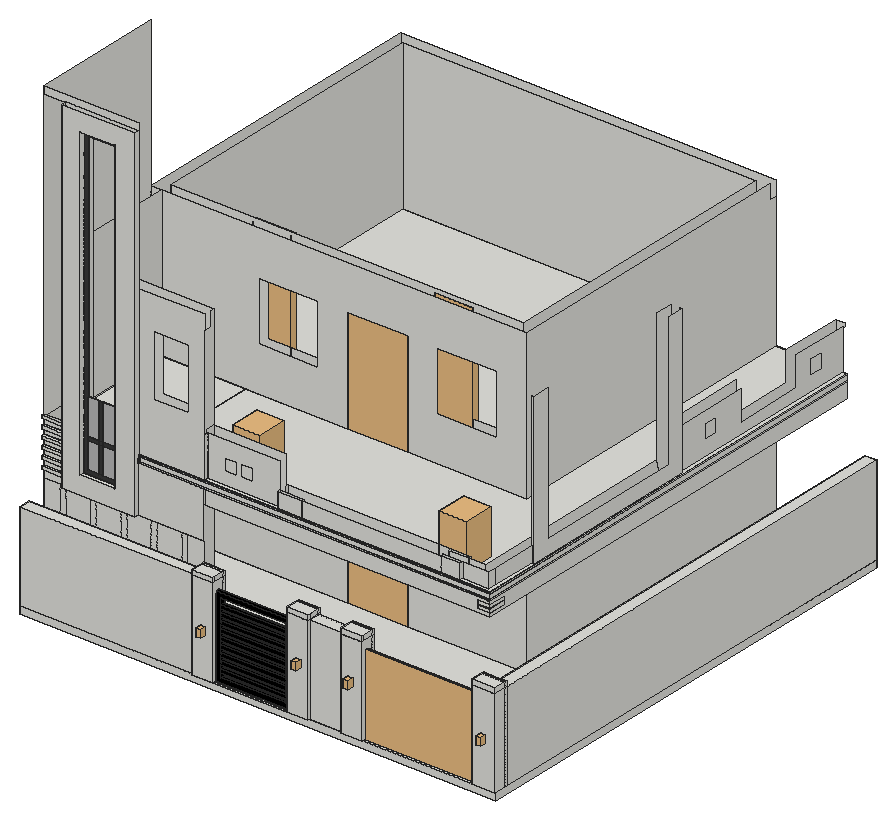
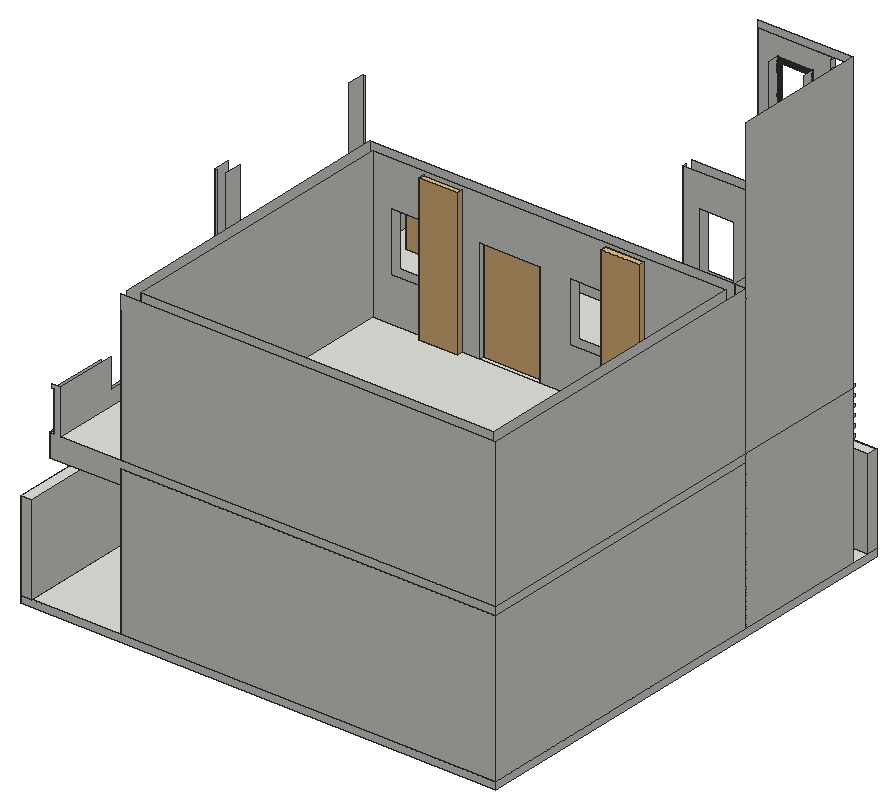
# SketchUp Ruby script. Lengths in inches.
U = 1.inch
M = Sketchup.active_model
def pt(a) = Geom::Point3d.new(a.map { |v| v * U })
def face(e, loops, mat)
  f = e.add_face(loops[0].map { |a| pt(a) })
  loops[1..].each { |l| e.add_face(l.map { |a| pt(a) }).erase! }
  f.material = f.back_material = mat if mat
  f
end
# faces: each face lists its corners as indices into pts; further lists are holes
def faces(e, pts, list, mat = nil) = list.each { |f| face(e, (f[0].is_a?(Array) ? f : [f]).map { |l| l.map { |i| pts[i] } }, mat) }
# xy, xz, yz: faces in a plane at the given z, y or x. An outline is a flat list of corners, or four numbers for a rectangle; further outlines are holes
def ring(l) = l.size == 4 ? [[l[0], l[1]], [l[2], l[1]], [l[2], l[3]], [l[0], l[3]]] : l.each_slice(2).to_a
def flat(e, list, mat, &to3) = list.each { |f| face(e, (f[0].is_a?(Array) ? f : [f]).map { |l| ring(l).map { |u, v| to3.(u, v) } }, mat) }
def xy(e, z, list, mat = nil) = flat(e, list, mat) { |x, y| [x, y, z] }
def xz(e, y, list, mat = nil) = flat(e, list, mat) { |x, z| [x, y, z] }
def yz(e, x, list, mat = nil) = flat(e, list, mat) { |y, z| [x, y, z] }
def lines(e, pts, list) = list.each { |a, b| e.add_line(pt(pts[a]), pt(pts[b])) }
# prism: a flat outline (further loops are holes) pulled along v
def prism(e, loops, v, mat = nil)
  f = face(e, loops, mat); d = Geom::Vector3d.new(v.map { |x| x * U })
  f.pushpull(f.normal.samedirection?(d) ? d.length : -d.length)
end
def box(e, o, s, mat = nil) = prism(e, [[o, [o[0] + s[0], o[1], o[2]], [o[0] + s[0], o[1] + s[1], o[2]], [o[0], o[1] + s[1], o[2]]]], [0, 0, s[2]], mat)
def at(x, y, z, deg = 0) = Geom::Transformation.translation(pt([x, y, z])) * Geom::Transformation.rotation(ORIGIN, Z_AXIS, deg.degrees)
def axes(o, x, y, z) = Geom::Transformation.new([*x, 0, *y, 0, *z, 0, *pt(o).to_a, 1])
def part(name) = M.definitions.add(name)
# library, detail: a bought-in or finely detailed component or shape, given as its bounding box
def library(name, o, s) = part(name).tap { |d| box(d.entities, o, s) }
def detail(e, o, s) = box(e.add_group.entities, o, s)
def put(e, d, t, mat = nil) = e.add_instance(d, t).tap { |i| i.material = mat if mat }
def group(e, t, mat = nil) = e.add_group.tap { |g| g.transformation = t; g.material = mat if mat }.entities
root = M.entities
M.materials.add("[Color M07]").color = [58, 58, 58]
M.materials.add("[Color M09]").color = [0, 0, 0]
M.materials.add("[Mirror 01]").color = [185, 185, 185]
c1 = library("Modern Gate 1",[0,0,0],[118.11,1.97,78.74])
c2 = library("Curtains 004",[-15.59,-2.26,0],[31.18,4.52,116.91])
c3 = library("Door 243 053",[-21.6,-2.79,-0.07],[43.2,5.58,82.64])
c4 = library("Lamp Wall Outdoor 94-02",[-1.89,-4.65,-3.17],[3.78,4.65,6.35])
c5 = library("Window 46-10",[-43.56,-2.12,0],[87.13,4.27,82.67])
c6 = library("Ficus elastica Belize 002",[-7.92,-8.8125,0.01],[22.14,24.73,36.43])
xy(root,-6,[[7.9375,1.1875,391.9375,385.1875]])
xy(root,0,[[147.375,0,164.42,1.1875],[164.42,0,224.25,1.1875],[224.25,0,241.3,1.1875],[267.83,0,284.875,1.1875],[373.38,0,391.9375,1.1875],
  [7.9375,1.1875,147.375,10.1875],[147.375,1.1875,164.42,10.1875],[164.42,1.1875,224.25,3.2],[224.25,1.1875,241.3,10.1875],[241.3,1.1875,267.83,10.1875],
  [267.83,1.1875,284.875,10.1875],[284.875,1.1875,373.38,10.1875],[373.38,1.1875,391.9375,10.1875],[164.42,3.2,224.25,6.14],[164.42,6.14,224.25,10.1875],
  [7.9375,10.1875,147.375,10.1875,147.375,11.875,164.42,11.875,164.42,10.1875,224.25,10.1875,224.25,11.875,241.3,11.875,241.3,10.1875,267.83,10.1875,267.83,11.875,284.875,11.875,284.875,10.1875,373.38,10.1875,373.38,11.875,382.9375,11.875,382.9375,385.1875,310.9375,385.1875,310.9375,133.1875,214.9375,133.1875,214.9375,142.1875,166.9375,142.1875,166.9375,133.1875,16.9375,133.1875,16.9375,34.1875,137.39,34.1875,137.39,25.1875,7.9375,25.1875],[147.375,10.1875,164.42,11.875],[224.25,10.1875,241.3,11.875],[267.83,10.1875,284.875,11.875],[373.38,10.1875,382.9375,11.875],
  [382.9375,10.1875,391.9375,11.875],[382.9375,11.875,391.9375,385.1875],[7.9375,25.1875,16.9375,133.1875],[16.9375,25.1875,137.39,34.1875],[7.9375,133.1875,166.9375,133.1875,166.9375,142.1875,16.9375,142.1875,16.9375,376.1875,301.9375,376.1875,301.9375,142.1875,214.9375,142.1875,214.9375,133.1875,310.9375,133.1875,310.9375,385.1875,7.9375,385.1875],
  [16.9375,142.1875,301.9375,376.1875],[16.9375,142.1875,301.9375,376.1875]])
xy(root,3.64,[[168.07,3.2,220.61,6.14]],"[Color M09]")
xy(root,6.82,[[168.07,3.2,220.61,6.14]],"[Color M09]")
xy(root,9.91,[[168.07,3.2,220.61,6.14]],"[Color M09]")
xy(root,12.64,[[168.07,3.2,220.61,6.14]],"[Color M09]")
xy(root,15.73,[[168.07,3.2,220.61,6.14]],"[Color M09]")
xy(root,18.46,[[168.07,3.2,220.61,6.14]],"[Color M09]")
xy(root,21.55,[[168.07,3.2,220.61,6.14]],"[Color M09]")
xy(root,24.29,[[168.07,3.2,220.61,6.14]],"[Color M09]")
xy(root,27.37,[[168.07,3.2,220.61,6.14]],"[Color M09]")
xy(root,30.11,[[168.07,3.2,220.61,6.14]],"[Color M09]")
xy(root,33.1875,[[168.07,3.2,220.61,6.14]],"[Color M09]")
xy(root,35.93,[[168.07,3.2,220.61,6.14]],"[Color M09]")
xy(root,36,[[94.9375,133.1875,142.9375,142.1875],[238.9375,133.1875,286.9375,142.1875]])
xy(root,39.01,[[168.07,3.2,220.61,6.14]],"[Color M09]")
xy(root,41.75,[[168.07,3.2,220.61,6.14]],"[Color M09]")
xy(root,44.83,[[168.07,3.2,220.61,6.14]],"[Color M09]")
xy(root,47.57,[[168.07,3.2,220.61,6.14]],"[Color M09]")
xy(root,50.65,[[168.07,3.2,220.61,6.14]],"[Color M09]")
xy(root,53.39,[[168.07,3.2,220.61,6.14]],"[Color M09]")
xy(root,56.47,[[168.07,3.2,220.61,6.14]],"[Color M09]")
xy(root,61.61,[[168.07,3.2,220.61,6.14]],"[Color M09]")
xy(root,65.25,[[164.42,3.2,224.25,6.14]],"[Color M09]")
xy(root,72,[[147.375,0,164.42,10.1875],[224.25,0,241.3,10.1875],[267.83,0,284.875,10.1875],[373.38,0,391.9375,10.1875],[7.9375,1.1875,147.375,10.1875],
  [241.3,1.1875,267.83,10.1875],[147.375,10.1875,164.42,11.875],[224.25,10.1875,241.3,11.875],[267.83,10.1875,284.875,11.875],[373.38,10.1875,382.9375,11.875],
  [382.9375,10.1875,391.9375,11.875],[382.9375,11.875,391.9375,385.1875]])
xy(root,75.875,[[147.375,0,164.42,10.1875],[224.25,0,241.3,10.1875],[267.83,0,284.875,10.1875],[373.38,0,391.9375,10.1875],[147.375,10.1875,164.42,11.875],
  [224.25,10.1875,241.3,11.875],[267.83,10.1875,284.875,11.875],[373.38,10.1875,382.9375,11.875],[382.9375,10.1875,391.9375,11.875]])
xy(root,82.42,[[25.22,21.625,84.16,25.1875],[84.16,24.75,137.39,25.1875]])
xy(root,84,[[94.9375,133.1875,142.9375,142.1875],[166.9375,133.1875,214.9375,142.1875],[238.9375,133.1875,286.9375,142.1875]])
xy(root,89.57,[[7.9375,22.625,25.22,25.1875]])
xy(root,91.92,[[7.9375,22.625,25.22,25.1875]])
xy(root,96.94,[[7.9375,22.625,25.22,25.1875]])
xy(root,97.01,[[39.8125,21.625,68,25.1875],[39.8125,26.1875,68,34.1875]])
xy(root,97.01,[[39.8125,25.1875,68,26.1875]],"[Color M07]")
xy(root,99.29,[[7.9375,22.625,25.22,25.1875]])
xy(root,100.22,[[52.28,25.1875,55.28,25.6875],[43.02,25.6875,52.28,26.1875],[52.28,25.6875,55.28,26.1875],[55.28,25.6875,64.8,26.1875]])
xy(root,100.22,[[43.02,25.1875,52.28,25.6875],[55.28,25.1875,64.8,25.6875]],"[Color M07]")
xy(root,104.32,[[7.9375,22.625,25.22,25.1875]])
xy(root,106.67,[[7.9375,22.625,25.22,25.1875]])
xy(root,108,[[137.39,25.1875,137.39,31.1875,361.9375,31.1875,361.9375,385.1875,367.9375,385.1875,367.9375,25.1875],[310.9375,379.1875,361.9375,385.1875]])
xy(root,111.31,[[358.4375,24.8125,368.3125,25.1875],[367.9375,25.1875,368.3125,38.6875]])
xy(root,111.69,[[7.9375,22.625,25.22,25.1875]])
xy(root,113.56,[[358.4375,24.8125,368.3125,25.1875],[367.9375,25.1875,368.3125,38.6875]])
xy(root,114.04,[[7.9375,22.625,25.22,25.1875]])
xy(root,114.61,[[358.4375,24.8125,368.3125,25.1875],[367.9375,25.1875,368.3125,38.6875]])
xy(root,116.86,[[358.4375,24.8125,368.3125,25.1875],[367.9375,25.1875,368.3125,38.6875]])
xy(root,119.07,[[7.9375,22.625,25.22,25.1875]])
xy(root,120,[[84.16,24.75,84.23,25.1875],[84.23,24.75,137.39,34.1875],[137.39,24.75,137.39,25.1875,367.9375,25.1875,367.9375,385.1875,368.375,385.1875,368.375,24.75],[137.39,31.1875,137.39,34.1875,84.23,34.1875,84.23,133.1875,310.9375,133.1875,310.9375,379.1875,361.9375,379.1875,361.9375,31.1875],[16.9375,34.1875,84.23,133.1875],
  [[7.9375,133.1875,310.9375,385.1875],[16.9375,142.1875,301.9375,376.1875]]])
xy(root,121,[[85.23,24.75,366.9375,25.1875],[366.9375,24.75,368.375,25.1875],[367.9375,25.1875,368.375,385.1875]])
xy(root,121.42,[[7.9375,22.625,25.22,25.1875]])
xy(root,121.86,[[52.28,25.1875,55.28,25.6875],[43.02,25.6875,52.28,26.1875],[52.28,25.6875,55.28,26.1875],[55.28,25.6875,64.8,26.1875]])
xy(root,121.86,[[43.02,25.1875,52.28,25.6875],[55.28,25.1875,64.8,25.6875]],"[Color M07]")
xy(root,124.49,[[52.28,25.1875,55.28,25.6875],[43.02,25.6875,52.28,26.1875],[52.28,25.6875,55.28,26.1875],[55.28,25.6875,64.8,26.1875]])
xy(root,124.49,[[43.02,25.1875,52.28,25.6875],[55.28,25.1875,64.8,25.6875]],"[Color M07]")
xy(root,125,[[85.23,24.75,366.9375,25.1875],[366.9375,24.75,368.375,25.1875],[367.9375,25.1875,368.375,385.1875]])
xy(root,126,[[84.23,24.75,85.23,25.1875],[85.23,24.75,368.375,24.75,368.375,385.1875,367.9375,385.1875,367.9375,25.1875,85.23,25.1875],[84.23,25.1875,137.39,34.1875],[137.39,25.1875,367.9375,25.1875,367.9375,385.1875,364.9375,385.1875,364.9375,220.375,367,220.375,367,70.91,364.9375,70.91,364.9375,28.1875,343.4,28.1875,343.4,25.625,196.07,25.625,196.07,28.1875,137.39,28.1875],[215.37,25.625,327.58,28.1875],
  [16.9375,34.1875,84.23,133.1875],[84.23,34.1875,196.07,34.1875,196.07,36.25,343.4,36.25,343.4,34.1875,357.6875,34.1875,357.6875,220.375,358.9375,220.375,358.9375,385.1875,310.9375,385.1875,310.9375,133.1875,214.9375,133.1875,214.9375,142.1875,166.9375,142.1875,166.9375,133.1875,84.23,133.1875],[196.07,34.1875,327.58,36.25],[7.9375,133.1875,166.9375,133.1875,166.9375,142.1875,16.9375,142.1875,16.9375,376.1875,301.9375,376.1875,301.9375,142.1875,214.9375,142.1875,214.9375,133.1875,310.9375,133.1875,310.9375,385.1875,7.9375,385.1875],[16.9375,142.1875,301.9375,376.1875]])
xy(root,126.44,[[7.9375,22.625,25.22,25.1875]])
xz(root,0,[[147.375,0,164.42,72],[224.25,0,241.3,72],[267.83,0,284.875,72],[373.38,0,391.9375,72],[147.375,72,164.42,75.875],
  [224.25,72,241.3,75.875],[267.83,72,284.875,75.875],[373.38,72,391.9375,75.875]])
xz(root,1.1875,[[7.9375,-6,391.9375,0],[7.9375,0,147.375,72],[241.3,0,267.83,72]])
xz(root,3.2,[[[164.42,0,224.25,65.25],[168.07,3.64,220.61,61.61]],[168.07,6.82,220.61,9.91],[168.07,12.64,220.61,15.73],[168.07,18.46,220.61,21.55],[168.07,24.29,220.61,27.37],
  [168.07,30.11,220.61,33.1875],[168.07,35.93,220.61,39.01],[168.07,41.75,220.61,44.83],[168.07,47.57,220.61,50.65],[168.07,53.39,220.61,56.47]],"[Color M09]")
xz(root,6.14,[[[164.42,0,224.25,65.25],[168.07,56.47,220.61,61.61],[168.07,3.64,220.61,6.82],[168.07,9.91,220.61,12.64],[168.07,50.65,220.61,53.39],[168.07,44.83,220.61,47.57],[168.07,39.01,220.61,41.75],[168.07,33.1875,220.61,35.93],[168.07,27.37,220.61,30.11],[168.07,21.55,220.61,24.29],[168.07,15.73,220.61,18.46]]],"[Color M09]")
xz(root,10.1875,[[7.9375,0,164.42,72],[224.25,0,284.875,72],[373.38,0,382.9375,72],[382.9375,0,391.9375,72],[147.375,72,164.42,75.875],
  [224.25,72,241.3,75.875],[267.83,72,284.875,75.875],[373.38,72,382.9375,75.875],[382.9375,72,391.9375,75.875]])
xz(root,11.875,[[147.375,0,164.42,72],[224.25,0,241.3,72],[267.83,0,284.875,72],[373.38,0,391.9375,72],[147.375,72,164.42,75.875],
  [224.25,72,241.3,75.875],[267.83,72,284.875,75.875],[373.38,72,382.9375,75.875],[382.9375,72,391.9375,75.875]])
xz(root,21.625,[[[25.22,82.42,84.16,359.98],[39.8125,97.01,68,345.39]]])
xz(root,22.625,[[7.9375,89.57,25.22,91.92],[7.9375,96.94,25.22,99.29],[7.9375,104.32,25.22,106.67],[7.9375,111.69,25.22,114.04],[7.9375,119.07,25.22,121.42],
  [7.9375,126.44,25.22,128.79]])
xz(root,24.75,[[84.16,82.42,137.39,120],[84.23,120,368.375,120,368.375,121,85.23,121,85.23,125,368.375,125,368.375,126,84.23,126]])
xz(root,24.8125,[[358.4375,111.31,368.3125,113.56],[358.4375,114.61,368.3125,116.86]])
xz(root,25.1875,[[7.9375,0,20.7,82.42],[20.7,0,25.22,82.42],[25.22,0,45.26,82.42],[45.26,0,49.78,82.42],[49.78,0,69.82,82.42],
  [69.82,0,74.35,82.42],[74.35,0,94.38,82.42],[94.38,0,98.91,82.42],[98.91,0,118.95,82.42],[118.95,0,123.47,82.42],
  [123.47,0,137.39,82.42],[7.9375,82.42,25.22,89.57],[[25.22,82.42,84.16,359.98],[39.8125,97.01,68,345.39]],[7.9375,89.57,25.22,91.92],[7.9375,91.92,25.22,96.94],
  [7.9375,96.94,25.22,99.29],[7.9375,99.29,25.22,104.32],[7.9375,104.32,25.22,106.67],[7.9375,106.67,25.22,111.69],[137.39,108,367.9375,108,367.9375,111.31,358.4375,111.31,358.4375,113.56,367.9375,113.56,367.9375,114.61,358.4375,114.61,358.4375,116.86,367.9375,116.86,367.9375,120,137.39,120],
  [7.9375,111.69,25.22,114.04],[7.9375,114.04,25.22,119.07],[7.9375,119.07,25.22,121.42],[[84.16,120,84.23,120,84.23,126,137.39,126,137.39,246,84.23,246,84.23,366,7.9375,366,7.9375,359.98,84.16,359.98],[96.26,169.96,124.63,219.71]],[85.23,121,367.9375,125],
  [7.9375,121.42,25.22,126.44],[7.9375,126.44,25.22,128.79]])
xz(root,25.1875,[[[39.8125,97.01,68,345.39],[43.02,100.22,64.8,342.18]],[52.28,100.22,55.28,121.86],[43.02,121.86,52.28,124.49],[52.28,121.86,55.28,124.49],[55.28,121.86,64.8,124.49],
  [52.28,124.49,55.28,153.17]],"[Color M07]")
xz(root,25.625,[[196.07,126,215.37,138],[215.37,126,327.58,138],[327.58,126,343.4,138]])
xz(root,25.6875,[[52.28,100.22,55.28,121.86],[43.02,121.86,52.28,124.49],[52.28,121.86,55.28,124.49],[55.28,121.86,64.8,124.49],[52.28,124.49,55.28,153.17]])
xz(root,25.6875,[[43.02,100.22,52.28,121.86],[55.28,100.22,64.8,121.86],[43.02,124.49,52.28,153.17],[55.28,124.49,64.8,153.17]],"[Mirror 01]")
xz(root,26.1875,[[[39.8125,97.01,68,345.39],[43.02,100.22,64.8,342.18]],[52.28,100.22,55.28,121.86],[43.02,121.86,52.28,124.49],[52.28,121.86,55.28,124.49],[55.28,121.86,64.8,124.49],
  [52.28,124.49,55.28,153.17]],"[Color M07]")
xz(root,26.1875,[[43.02,100.22,52.28,121.86],[55.28,100.22,64.8,121.86],[43.02,124.49,52.28,153.17],[55.28,124.49,64.8,153.17]],"[Mirror 01]")
xz(root,28.1875,[[[137.39,126,196.07,159],[151.84,136.53,161.34,146.03],[164.22,136.53,173.72,146.03]],[196.07,126,215.37,138],[327.58,126,343.4,138],[343.4,126,364.9375,138]])
xz(root,31.1875,[[137.39,108,361.9375,120]])
xz(root,34.1875,[[16.9375,0,16.9375,120,39.8125,120,39.8125,97.01,68,97.01,68,120,137.39,120,137.39,0],[16.9375,120,39.8125,126],[39.8125,120,68,126],[68,120,84.23,126],[16.9375,126,39.8125,246],
  [[68,126,137.39,246],[96.26,169.96,124.63,219.71]],[137.39,126,196.07,162],[327.58,126,343.4,138],[343.4,126,357.6875,138]])
xz(root,36.25,[[196.07,126,327.58,138],[327.58,126,343.4,138]])
xz(root,38.6875,[[367.9375,111.31,368.3125,113.56],[367.9375,114.61,368.3125,116.86]])
xz(root,70.91,[[364.9375,126,367,247]])
xz(root,133.1875,[[7.9375,0,16.9375,120],[[16.9375,0,166.9375,0,166.9375,84,214.9375,84,214.9375,0,310.9375,0,310.9375,120,16.9375,120],[94.9375,36,142.9375,84],[238.9375,36,286.9375,84]],[7.9375,120,16.9375,126],[16.9375,120,84.23,126],[7.9375,126,16.9375,246],
  [[16.9375,126,166.9375,126,166.9375,210,214.9375,210,214.9375,126,310.9375,126,310.9375,246,16.9375,246],[94.9375,162,142.9375,210],[238.9375,162,286.9375,210]]])
xz(root,142.1875,[[[16.9375,0,16.9375,120,301.9375,120,301.9375,0,214.9375,0,214.9375,84,166.9375,84,166.9375,0],[94.9375,36,142.9375,84],[238.9375,36,286.9375,84]],[[16.9375,126,16.9375,246,301.9375,246,301.9375,126,214.9375,126,214.9375,210,166.9375,210,166.9375,126],[94.9375,162,142.9375,210],[238.9375,162,286.9375,210]]])
xz(root,220.375,[[357.6875,126,358.9375,138],[364.9375,126,364.9375,159,366.3125,159,366.3125,162,364.9375,162,364.9375,244.8125,367,244.8125,367,126]])
xz(root,376.1875,[[16.9375,0,301.9375,120],[16.9375,126,301.9375,246]])
xz(root,379.1875,[[310.9375,108,361.9375,120]])
xz(root,385.1875,[[7.9375,-6,391.9375,0],[7.9375,0,310.9375,120],[382.9375,0,391.9375,72],[310.9375,108,310.9375,120,7.9375,120,7.9375,126,358.9375,126,358.9375,162,366.3125,162,366.3125,159,364.9375,159,364.9375,126,367.9375,126,367.9375,108],[367.9375,120,368.375,121],
  [367.9375,125,368.375,126],[7.9375,126,310.9375,246]])
yz(root,7.9375,[[1.1875,-6,385.1875,0],[1.1875,0,10.1875,72],[25.1875,0,133.1875,126],[133.1875,0,385.1875,120],[22.625,89.57,25.1875,91.92],
  [22.625,96.94,25.1875,99.29],[22.625,104.32,25.1875,106.67],[22.625,111.69,25.1875,114.04],[22.625,119.07,25.1875,121.42],[133.1875,120,385.1875,126],
  [25.1875,126,133.1875,366],[133.1875,126,385.1875,246],[22.625,126.44,25.1875,128.79]])
yz(root,16.9375,[[34.1875,0,133.1875,120],[142.1875,0,376.1875,120],[34.1875,120,133.1875,126],[34.1875,126,133.1875,246],[142.1875,126,376.1875,246]])
yz(root,25.22,[[21.625,82.42,21.625,359.98,22.5,359.98,22.5,357.63,25.1875,357.63,25.1875,351.6,22.5,351.6,22.5,349.25,25.1875,349.25,25.1875,341.29,22.5,341.29,22.5,338.94,25.1875,338.94,25.1875,331.1,22.5,331.1,22.5,328.75,25.1875,328.75,25.1875,320.92,22.5,320.92,22.5,318.57,25.1875,318.57,25.1875,310.73,22.5,310.73,22.5,308.38,25.1875,308.38,25.1875,300.54,22.5,300.54,22.5,298.19,25.1875,298.19,25.1875,290.35,22.5,290.35,22.5,288,25.1875,288,25.1875,280.17,22.5,280.17,22.5,277.82,25.1875,277.82,25.1875,269.98,22.5,269.98,22.5,267.63,25.1875,267.63,25.1875,259.79,22.5,259.79,22.5,257.44,25.1875,257.44,25.1875,249.6,22.5,249.6,22.5,247.25,25.1875,247.25,25.1875,239.42,22.5,239.42,22.5,237.07,25.1875,237.07,25.1875,232.04,22.5,232.04,22.5,229.69,25.1875,229.69,25.1875,224.67,22.625,224.67,22.625,222.32,25.1875,222.32,25.1875,217.29,22.625,217.29,22.625,214.94,25.1875,214.94,25.1875,209.92,22.625,209.92,22.625,207.57,25.1875,207.57,25.1875,202.54,22.625,202.54,22.625,200.19,25.1875,200.19,25.1875,195.17,22.625,195.17,22.625,192.82,25.1875,192.82,25.1875,187.79,22.5,187.79,22.5,185.44,25.1875,185.44,25.1875,180.42,22.5,180.42,22.5,178.07,25.1875,178.07,25.1875,173.04,22.5,173.04,22.5,170.69,25.1875,170.69,25.1875,165.67,22.5,165.67,22.5,163.32,25.1875,163.32,25.1875,158.29,22.5,158.29,22.5,155.94,25.1875,155.94,25.1875,150.92,22.5,150.92,22.5,148.57,25.1875,148.57,25.1875,143.54,22.625,143.54,22.625,141.19,25.1875,141.19,25.1875,136.17,22.625,136.17,22.625,133.82,25.1875,133.82,25.1875,128.79,22.625,128.79,22.625,126.44,25.1875,126.44,25.1875,121.42,22.625,121.42,22.625,119.07,25.1875,119.07,25.1875,114.04,22.625,114.04,22.625,111.69,25.1875,111.69,25.1875,106.67,22.625,106.67,22.625,104.32,25.1875,104.32,25.1875,99.29,22.625,99.29,22.625,96.94,25.1875,96.94,25.1875,91.92,22.625,91.92,22.625,89.57,25.1875,89.57,25.1875,82.42],[22.625,89.57,25.1875,91.92],[22.625,96.94,25.1875,99.29],[22.625,104.32,25.1875,106.67],[22.625,111.69,25.1875,114.04],
  [22.625,119.07,25.1875,121.42],[22.625,126.44,25.1875,128.79]])
yz(root,39.8125,[[21.625,97.01,25.1875,345.39],[26.1875,97.01,34.1875,345.39]])
yz(root,39.8125,[[25.1875,97.01,26.1875,345.39]],"[Color M07]")
yz(root,43.02,[[25.6875,100.22,26.1875,121.86],[25.1875,121.86,25.6875,124.49],[25.6875,121.86,26.1875,124.49],[25.6875,124.49,26.1875,153.17]])
yz(root,43.02,[[25.1875,100.22,25.6875,121.86],[25.1875,124.49,25.6875,153.17]],"[Color M07]")
yz(root,52.28,[[25.6875,100.22,26.1875,121.86],[25.1875,121.86,25.6875,124.49],[25.6875,121.86,26.1875,124.49],[25.6875,124.49,26.1875,153.17]])
yz(root,52.28,[[25.1875,100.22,25.6875,121.86],[25.1875,124.49,25.6875,153.17]],"[Color M07]")
yz(root,55.28,[[25.6875,100.22,26.1875,121.86],[25.1875,121.86,25.6875,124.49],[25.6875,121.86,26.1875,124.49],[25.6875,124.49,26.1875,153.17]])
yz(root,55.28,[[25.1875,100.22,25.6875,121.86],[25.1875,124.49,25.6875,153.17]],"[Color M07]")
yz(root,64.8,[[25.6875,100.22,26.1875,121.86],[25.1875,121.86,25.6875,124.49],[25.6875,121.86,26.1875,124.49],[25.6875,124.49,26.1875,153.17]])
yz(root,64.8,[[25.1875,100.22,25.6875,121.86],[25.1875,124.49,25.6875,153.17]],"[Color M07]")
yz(root,68,[[21.625,97.01,25.1875,345.39],[26.1875,97.01,34.1875,345.39]])
yz(root,68,[[25.1875,97.01,26.1875,345.39]],"[Color M07]")
yz(root,84.16,[[21.625,82.42,24.75,82.42,24.75,120,25.1875,120,25.1875,359.98,21.625,359.98],[24.75,82.42,25.1875,120]])
yz(root,84.23,[[24.75,120,25.1875,125],[25.1875,120,34.1875,126],[34.1875,120,133.1875,126],[24.75,125,25.1875,126]])
yz(root,85.23,[[24.75,121,25.1875,125]])
yz(root,94.9375,[[133.1875,36,142.1875,84]])
yz(root,137.39,[[25.1875,0,34.1875,0,34.1875,120,31.1875,120,31.1875,108,24.75,108,24.75,82.42,25.1875,82.42],[24.75,108,25.1875,120],[25.1875,108,31.1875,120],[25.1875,126,28.1875,126,28.1875,159,26.8125,159,26.8125,162,34.1875,162,34.1875,246,31.1875,246,31.1875,234,25.1875,234],[28.1875,126,34.1875,126,34.1875,162,26.8125,162,26.8125,159,28.1875,159]])
yz(root,142.9375,[[133.1875,36,142.1875,84]])
yz(root,147.375,[[0,0,1.1875,72],[1.1875,0,11.875,72],[0,72,1.1875,75.875],[1.1875,72,10.1875,75.875],[10.1875,72,11.875,75.875]])
yz(root,164.42,[[0,0,3.2,0,3.2,65.25,6.14,65.25,6.14,0,10.1875,0,10.1875,72,0,72],[10.1875,0,11.875,72],[0,72,1.1875,75.875],[1.1875,72,10.1875,75.875],[10.1875,72,11.875,75.875]])
yz(root,164.42,[[3.2,0,6.14,65.25]],"[Color M09]")
yz(root,166.9375,[[133.1875,0,142.1875,84],[133.1875,126,142.1875,210]])
yz(root,168.07,[[3.2,3.64,6.14,6.82],[3.2,9.91,6.14,12.64],[3.2,15.73,6.14,18.46],[3.2,21.55,6.14,24.29],[3.2,27.37,6.14,30.11],
  [3.2,33.1875,6.14,35.93],[3.2,39.01,6.14,41.75],[3.2,44.83,6.14,47.57],[3.2,50.65,6.14,53.39],[3.2,56.47,6.14,61.61]],"[Color M09]")
yz(root,196.07,[[25.625,126,28.1875,138],[34.1875,126,36.25,138]])
yz(root,214.9375,[[133.1875,0,142.1875,84],[133.1875,126,142.1875,210]])
yz(root,215.37,[[25.625,126,28.1875,138]])
yz(root,220.61,[[3.2,3.64,6.14,6.82],[3.2,9.91,6.14,12.64],[3.2,15.73,6.14,18.46],[3.2,21.55,6.14,24.29],[3.2,27.37,6.14,30.11],
  [3.2,33.1875,6.14,35.93],[3.2,39.01,6.14,41.75],[3.2,44.83,6.14,47.57],[3.2,50.65,6.14,53.39],[3.2,56.47,6.14,61.61]],"[Color M09]")
yz(root,224.25,[[0,0,0,72,10.1875,72,10.1875,0,6.14,0,6.14,65.25,3.2,65.25,3.2,0],[10.1875,0,11.875,72],[0,72,1.1875,75.875],[1.1875,72,10.1875,75.875],[10.1875,72,11.875,75.875]])
yz(root,224.25,[[3.2,0,6.14,65.25]],"[Color M09]")
yz(root,238.9375,[[133.1875,36,142.1875,84]])
yz(root,241.3,[[0,0,1.1875,72],[1.1875,0,11.875,72],[0,72,1.1875,75.875],[1.1875,72,10.1875,75.875],[10.1875,72,11.875,75.875]])
yz(root,267.83,[[0,0,1.1875,72],[1.1875,0,11.875,72],[0,72,1.1875,75.875],[1.1875,72,10.1875,75.875],[10.1875,72,11.875,75.875]])
yz(root,284.875,[[0,0,10.1875,72],[10.1875,0,11.875,72],[0,72,1.1875,75.875],[1.1875,72,10.1875,75.875],[10.1875,72,11.875,75.875]])
yz(root,286.9375,[[133.1875,36,142.1875,84]])
yz(root,301.9375,[[142.1875,0,376.1875,120],[142.1875,126,376.1875,246]])
yz(root,310.9375,[[133.1875,0,385.1875,0,385.1875,108,379.1875,108,379.1875,120,133.1875,120],[379.1875,108,385.1875,120],[133.1875,126,385.1875,126,385.1875,234,379.1875,234,379.1875,246,133.1875,246]])
yz(root,327.58,[[34.1875,126,36.25,138]])
yz(root,343.4,[[25.625,126,28.1875,138],[34.1875,126,36.25,138]])
yz(root,357.6875,[[34.1875,126,34.1875,138,206.85,138,209.6875,126],[209.6875,126,206.85,138,206.85,244.8125,220.375,244.8125,220.375,126]])
yz(root,358.4375,[[24.8125,111.31,25.1875,113.56],[24.8125,114.61,25.1875,116.86]])
yz(root,358.9375,[[220.375,126,220.375,162,284.83,162,284.83,138,335.01,138,335.01,162,385.1875,162,385.1875,126]])
yz(root,361.9375,[[31.1875,108,379.1875,120]])
yz(root,364.9375,[[28.1875,126,34.1875,138],[34.1875,126,70.91,138],[[220.375,126,385.1875,126,385.1875,159,338.01,159,338.01,135,281.83,135,281.83,159,220.375,159],[351.9,138.13,363.65,149.88],[245.53,138.13,257.28,149.88]]])
yz(root,367,[[70.91,126,220.375,126,220.375,244.8125,206.85,244.8125,206.85,138,84.5,138,84.5,247,70.91,247]])
yz(root,367.9375,[[25.1875,108,385.1875,108,385.1875,120,25.1875,120,25.1875,116.86,38.6875,116.86,38.6875,114.61,25.1875,114.61,25.1875,113.56,38.6875,113.56,38.6875,111.31,25.1875,111.31],[25.1875,121,385.1875,125]])
yz(root,368.3125,[[24.8125,111.31,38.6875,113.56],[24.8125,114.61,38.6875,116.86]])
yz(root,368.375,[[24.75,120,385.1875,121],[24.75,125,385.1875,126]])
yz(root,373.38,[[0,0,10.1875,72],[10.1875,0,11.875,72],[0,72,1.1875,75.875],[1.1875,72,10.1875,75.875],[10.1875,72,11.875,75.875]])
yz(root,382.9375,[[10.1875,0,385.1875,72],[10.1875,72,11.875,75.875]])
yz(root,391.9375,[[1.1875,-6,385.1875,0],[0,0,10.1875,72],[10.1875,0,11.875,72],[11.875,0,385.1875,72],[0,72,10.1875,75.875],
  [10.1875,72,11.875,75.875]])
p = [[16.9375,25.1875,126],[16.9375,34.1875,126],[85.23,25.1875,126],[85.23,25.1875,125]]
lines(root,p,[[0,1],[2,3]])
put(root,c1,axes([284.875,3,0],[0.74934,0,0],[0,1,0],[0,0,0.83]))
put(root,c2,at(98.31,144.46,0))
put(root,c2,at(245.3125,144.22,0))
put(root,c3,axes([190.9375,135.97,0.07],[-1.11105,0,0],[0,-1,0],[0,0,1.01657]))
put(root,c2,at(138.86,144.45,3.09))
put(root,c2,at(279.9,144.45,3.09))
put(root,c4,at(156.35,0,35.14))
put(root,c4,at(382.38,0,36.48))
put(root,c4,at(233.2,0,38.43))
put(root,c5,axes([262.93,135.31,36],[0.5509,0,0],[0,1,0],[0,0,0.58062]))
put(root,c5,axes([118.93,135.31,36],[0.5509,0,0],[0,1,0],[0,0,0.58062]))
put(root,c4,at(275.08,0,39.94))
put(root,c2,at(98.31,144.46,126))
put(root,c2,at(245.3125,144.22,126))
put(root,c3,axes([190.9375,135.97,126.07],[-1.11105,0,0],[0,-1,0],[0,0,1.01657]))
put(root,c6,at(325.93,45.17,126))
put(root,c6,at(154.96,50.14,126))
